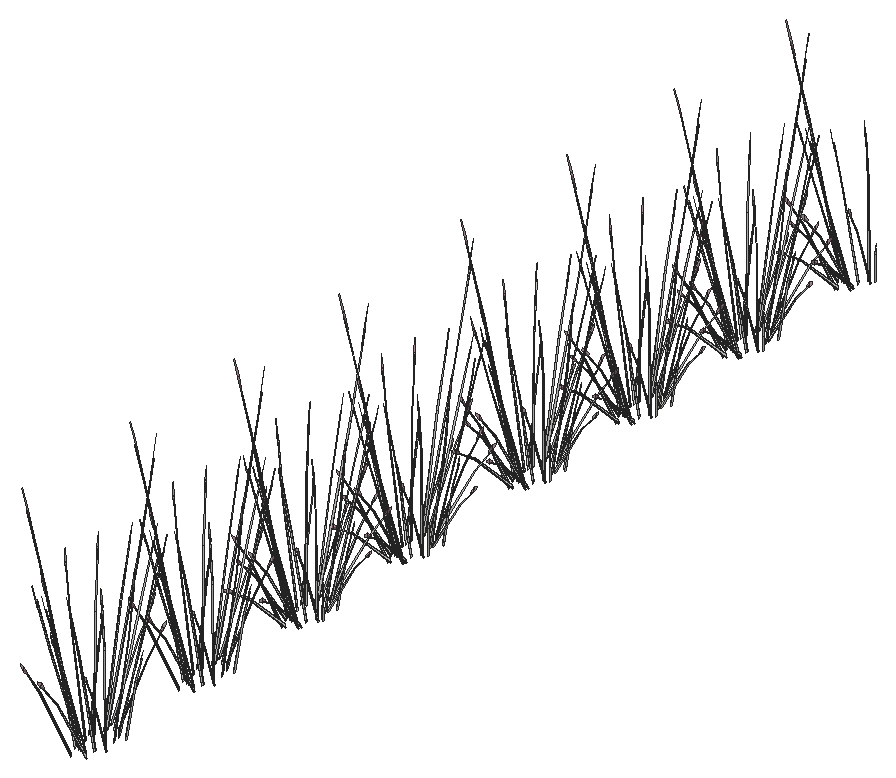
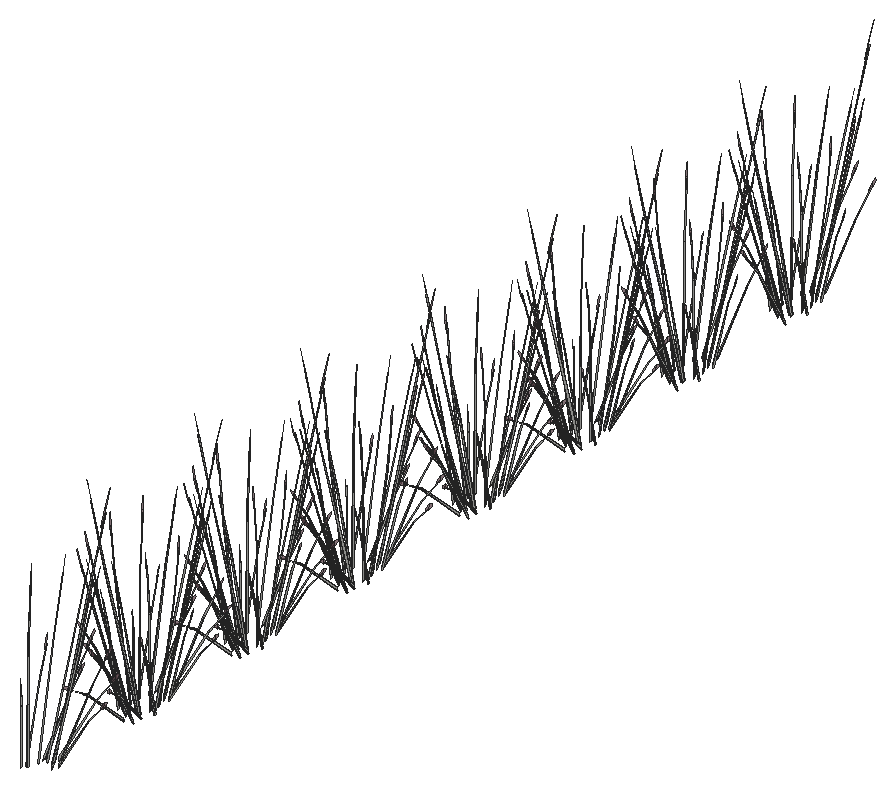
# SketchUp Ruby script. Lengths in inches.
U = 1.inch
M = Sketchup.active_model
def pt(a) = Geom::Point3d.new(a.map { |v| v * U })
def face(e, loops, mat)
  f = e.add_face(loops[0].map { |a| pt(a) })
  loops[1..].each { |l| e.add_face(l.map { |a| pt(a) }).erase! }
  f.material = f.back_material = mat if mat
  f
end
# faces: each face lists its corners as indices into pts; further lists are holes
def faces(e, pts, list, mat = nil) = list.each { |f| face(e, (f[0].is_a?(Array) ? f : [f]).map { |l| l.map { |i| pts[i] } }, mat) }
# xy, xz, yz: faces in a plane at the given z, y or x. An outline is a flat list of corners, or four numbers for a rectangle; further outlines are holes
def ring(l) = l.size == 4 ? [[l[0], l[1]], [l[2], l[1]], [l[2], l[3]], [l[0], l[3]]] : l.each_slice(2).to_a
def flat(e, list, mat, &to3) = list.each { |f| face(e, (f[0].is_a?(Array) ? f : [f]).map { |l| ring(l).map { |u, v| to3.(u, v) } }, mat) }
def xy(e, z, list, mat = nil) = flat(e, list, mat) { |x, y| [x, y, z] }
def xz(e, y, list, mat = nil) = flat(e, list, mat) { |x, z| [x, y, z] }
def yz(e, x, list, mat = nil) = flat(e, list, mat) { |y, z| [x, y, z] }
def lines(e, pts, list) = list.each { |a, b| e.add_line(pt(pts[a]), pt(pts[b])) }
# prism: a flat outline (further loops are holes) pulled along v
def prism(e, loops, v, mat = nil)
  f = face(e, loops, mat); d = Geom::Vector3d.new(v.map { |x| x * U })
  f.pushpull(f.normal.samedirection?(d) ? d.length : -d.length)
end
def box(e, o, s, mat = nil) = prism(e, [[o, [o[0] + s[0], o[1], o[2]], [o[0] + s[0], o[1] + s[1], o[2]], [o[0], o[1] + s[1], o[2]]]], [0, 0, s[2]], mat)
def at(x, y, z, deg = 0) = Geom::Transformation.translation(pt([x, y, z])) * Geom::Transformation.rotation(ORIGIN, Z_AXIS, deg.degrees)
def axes(o, x, y, z) = Geom::Transformation.new([*x, 0, *y, 0, *z, 0, *pt(o).to_a, 1])
def part(name) = M.definitions.add(name)
# library, detail: a bought-in or finely detailed component or shape, given as its bounding box
def library(name, o, s) = part(name).tap { |d| box(d.entities, o, s) }
def detail(e, o, s) = box(e.add_group.entities, o, s)
def put(e, d, t, mat = nil) = e.add_instance(d, t).tap { |i| i.material = mat if mat }
def group(e, t, mat = nil) = e.add_group.tap { |g| g.transformation = t; g.material = mat if mat }.entities
root = M.entities
M.materials.add("LightPink_Translucent").color = [144, 107, 117]
M.materials["LightPink_Translucent"].alpha = 0.75
c1 = part("blade")
p = [[2.15,0.21,22],[0,0.17,0],[0.09,0.45,0],[2.18,0.31,22],[2.29,0.31,22],[0.38,0.45,0],
  [2.48,0.24,33],[2.49,0.24,33],[2.48,0.22,33]]
faces(c1.entities,p,[[0,1,2,3],[4,5,2,3],[6,3,4,7],[8,0,3,6]])
c2 = part("seeds")
p = [[0.3,-0.1,1.38],[-0.01,-0.03,1.59],[-0.01,-0.03,0.03],[0.14,-0.07,-0.07],[0.29,-0.03,3],[0.15,0.01,3.11]]
faces(c2.entities,p,[[0,1,2,3],[1,0,4,5]],"LightPink_Translucent")
c3 = part("blade with seeds")
put(c3.entities,c1,at(0,0,0))
put(c3.entities,c2,axes([2.4,0.25,30.99],[1.5799,-0.05474,1.17369],[-0.12525,1.92788,0.29478],[-0.07173,-0.02425,1.56792]))
put(root,c3,axes([252.66,9.92,2.61],[-0.02599,0.0467,1.28742],[-0.25468,-0.15757,-0.12165],[-0.00922,-0.20381,0.22783]))
put(root,c3,axes([251.28,9.02,2.61],[-0.00478,0.07329,1.28742],[-0.23551,0.26599,-0.12165],[-0.0693,-0.13596,0.22783]))
put(root,c3,axes([251.9375,10.4,2.625],[0.1886,-0.20781,0.04667],[0.09231,0.37894,0.3674],[-0.01821,-0.16704,0.56022]))
put(root,c3,axes([251.29,10.46,2.625],[0.11633,-0.38842,0.04667],[0.16566,0.22614,0.3674],[-0.05356,-0.12453,0.56022]))
put(root,c3,axes([251.34,10.41,3.13],[-0.17082,0.58618,-0.09885],[-0.24738,-0.33771,-0.54865],[-0.08599,-0.16561,0.83366]))
put(root,c3,axes([252.51,11.0625,2.625],[0.21034,0.02849,0.04667],[-0.00577,0.43021,0.3674],[0.02201,-0.1648,0.56022]))
put(root,c3,axes([253.35,12.25,2.61],[-0.03343,-0.00464,1.28742],[-0.13883,-0.49759,-0.12165],[0.05575,-0.16361,0.22783]))
put(root,c3,axes([250.75,11.22,2.625],[0.01289,-0.46496,0.04667],[0.19462,0.01275,0.3674],[-0.07455,-0.04865,0.56022]))
put(root,c3,axes([252.86,12.27,2.625],[0.17571,0.25715,0.04667],[-0.1023,0.3662,0.3674],[0.05634,-0.11839,0.56022]))
put(root,c3,axes([250.48,10.61,2.61],[0.01898,0.06102,1.28742],[-0.09148,0.54852,-0.12165],[-0.09264,0.00397,0.22783]))
put(root,c3,axes([250.44,12.49,2.625],[-0.09401,-0.41691,0.04667],[0.17143,-0.20406,0.3674],[-0.07557,0.04026,0.56022]))
put(root,c3,axes([252.88,13.7,2.625],[0.09401,0.41691,0.04667],[-0.17143,0.20406,0.3674],[0.07557,-0.04026,0.56022]))
put(root,c3,axes([253.29,15.35,2.61],[-0.02314,-0.05353,1.28742],[0.05063,-0.5738,-0.12165],[0.09117,-0.03666,0.22783]))
put(root,c3,axes([250.47,13.91,2.625],[-0.17571,-0.25715,0.04667],[0.1023,-0.3662,0.3674],[-0.05634,0.11839,0.56022]))
put(root,c3,axes([249.81,13.61,2.61],[0.03267,0.0164,1.28742],[0.10105,0.54025,-0.12165],[-0.06687,0.1418,0.22783]))
put(root,c3,axes([252.58,14.96,2.625],[-0.01289,0.46496,0.04667],[-0.19462,-0.01275,0.3674],[0.07455,0.04865,0.56022]))
put(root,c3,axes([251.78,15.97,2.61],[0.00076,-0.07403,1.28742],[0.21935,-0.3266,-0.12165],[0.07619,0.11658,0.22783]))
put(root,c3,axes([250.82,15.12,2.625],[-0.21034,-0.02849,0.04667],[0.00577,-0.43021,0.3674],[-0.02201,0.1648,0.56022]))
put(root,c3,axes([252.04,15.73,2.625],[-0.11633,0.38842,0.04667],[-0.16566,-0.22614,0.3674],[0.05356,0.12453,0.56022]))
put(root,c3,axes([251.39,15.79,2.625],[-0.1886,0.20781,0.04667],[-0.09231,-0.37894,0.3674],[0.01821,0.16704,0.56022]))
put(root,c3,axes([250.86,14.92,3.11],[0.2813,0.0303,-0.09797],[-0.00769,0.57361,-0.54375],[-0.01954,0.22092,0.82622]))
put(root,c3,axes([250.27,16.43,2.61],[0.02904,-0.03692,1.28742],[0.24001,0.24555,-0.12165],[-0.00564,0.20445,0.22783]))
put(root,c3,axes([252.66,26.78,2.61],[-0.02599,0.0467,1.28742],[-0.25468,-0.15757,-0.12165],[-0.00922,-0.20381,0.22783]))
put(root,c3,axes([251.28,25.89,2.61],[-0.00478,0.07329,1.28742],[-0.23551,0.26599,-0.12165],[-0.0693,-0.13596,0.22783]))
put(root,c3,axes([251.9375,27.27,2.625],[0.1886,-0.20781,0.04667],[0.09231,0.37894,0.3674],[-0.01821,-0.16704,0.56022]))
put(root,c3,axes([251.29,27.32,2.625],[0.11633,-0.38842,0.04667],[0.16566,0.22614,0.3674],[-0.05356,-0.12453,0.56022]))
put(root,c3,axes([251.34,27.28,3.13],[-0.17082,0.58618,-0.09885],[-0.24738,-0.33771,-0.54865],[-0.08599,-0.16561,0.83366]))
put(root,c3,axes([252.51,27.93,2.625],[0.21034,0.02849,0.04667],[-0.00577,0.43021,0.3674],[0.02201,-0.1648,0.56022]))
put(root,c3,axes([253.35,29.12,2.61],[-0.03343,-0.00464,1.28742],[-0.13883,-0.49759,-0.12165],[0.05575,-0.16361,0.22783]))
put(root,c3,axes([250.75,28.09,2.625],[0.01289,-0.46496,0.04667],[0.19462,0.01275,0.3674],[-0.07455,-0.04865,0.56022]))
put(root,c3,axes([252.86,29.14,2.625],[0.17571,0.25715,0.04667],[-0.1023,0.3662,0.3674],[0.05634,-0.11839,0.56022]))
put(root,c3,axes([250.48,27.48,2.61],[0.01898,0.06102,1.28742],[-0.09148,0.54852,-0.12165],[-0.09264,0.00397,0.22783]))
put(root,c3,axes([250.44,29.35,2.625],[-0.09401,-0.41691,0.04667],[0.17143,-0.20406,0.3674],[-0.07557,0.04026,0.56022]))
put(root,c3,axes([252.88,30.57,2.625],[0.09401,0.41691,0.04667],[-0.17143,0.20406,0.3674],[0.07557,-0.04026,0.56022]))
put(root,c3,axes([253.29,32.22,2.61],[-0.02314,-0.05353,1.28742],[0.05063,-0.5738,-0.12165],[0.09117,-0.03666,0.22783]))
put(root,c3,axes([250.47,30.78,2.625],[-0.17571,-0.25715,0.04667],[0.1023,-0.3662,0.3674],[-0.05634,0.11839,0.56022]))
put(root,c3,axes([249.81,30.48,2.61],[0.03267,0.0164,1.28742],[0.10105,0.54025,-0.12165],[-0.06687,0.1418,0.22783]))
put(root,c3,axes([252.58,31.83,2.625],[-0.01289,0.46496,0.04667],[-0.19462,-0.01275,0.3674],[0.07455,0.04865,0.56022]))
put(root,c3,axes([251.78,32.84,2.61],[0.00076,-0.07403,1.28742],[0.21935,-0.3266,-0.12165],[0.07619,0.11658,0.22783]))
put(root,c3,axes([250.82,31.99,2.625],[-0.21034,-0.02849,0.04667],[0.00577,-0.43021,0.3674],[-0.02201,0.1648,0.56022]))
put(root,c3,axes([252.04,32.6,2.625],[-0.11633,0.38842,0.04667],[-0.16566,-0.22614,0.3674],[0.05356,0.12453,0.56022]))
put(root,c3,axes([251.39,32.65,2.625],[-0.1886,0.20781,0.04667],[-0.09231,-0.37894,0.3674],[0.01821,0.16704,0.56022]))
put(root,c3,axes([250.86,31.79,3.11],[0.2813,0.0303,-0.09797],[-0.00769,0.57361,-0.54375],[-0.01954,0.22092,0.82622]))
put(root,c3,axes([250.27,33.3,2.61],[0.02904,-0.03692,1.28742],[0.24001,0.24555,-0.12165],[-0.00564,0.20445,0.22783]))
put(root,c3,axes([251.55,42.32,2.61],[-0.03915,-0.08573,1.26972],[-0.26126,0.05435,-0.2008],[-0.0417,-0.20505,0.10183]))
put(root,c3,axes([252.72,43.375,2.61],[-0.00247,-0.12169,1.26972],[-0.20868,-0.35171,-0.2008],[0.03226,-0.2132,0.10183]))
put(root,c3,axes([252.66,42.9375,2.61],[-0.02599,0.0467,1.28742],[-0.25468,-0.15757,-0.12165],[-0.00922,-0.20381,0.22783]))
put(root,c3,axes([251.28,42.04,2.61],[-0.00478,0.07329,1.28742],[-0.23551,0.26599,-0.12165],[-0.0693,-0.13596,0.22783]))
put(root,c3,axes([251.9375,43.42,2.625],[0.1886,-0.20781,0.04667],[0.09231,0.37894,0.3674],[-0.01821,-0.16704,0.56022]))
put(root,c3,axes([251.29,43.48,2.625],[0.11633,-0.38842,0.04667],[0.16566,0.22614,0.3674],[-0.05356,-0.12453,0.56022]))
put(root,c3,axes([251.34,43.44,3.13],[-0.17082,0.58618,-0.09885],[-0.24738,-0.33771,-0.54865],[-0.08599,-0.16561,0.83366]))
put(root,c3,axes([252.51,44.08,2.625],[0.21034,0.02849,0.04667],[-0.00577,0.43021,0.3674],[0.02201,-0.1648,0.56022]))
put(root,c3,axes([250.6875,43.27,2.61],[-0.05507,-0.00432,1.26972],[-0.17533,0.4316,-0.2008],[-0.09355,-0.08819,0.10183]))
put(root,c3,axes([253.35,45.27,2.61],[-0.03343,-0.00464,1.28742],[-0.13883,-0.49759,-0.12165],[0.05575,-0.16361,0.22783]))
put(root,c3,axes([250.75,44.24,2.625],[0.01289,-0.46496,0.04667],[0.19462,0.01275,0.3674],[-0.07455,-0.04865,0.56022]))
put(root,c3,axes([252.86,45.29,2.625],[0.17571,0.25715,0.04667],[-0.1023,0.3662,0.3674],[0.05634,-0.11839,0.56022]))
put(root,c3,axes([253.48,45.86,2.61],[0.03552,-0.09314,1.26972],[-0.04546,-0.57131,-0.2008],[0.08912,-0.10832,0.10183]))
put(root,c3,axes([250.48,43.63,2.61],[0.01898,0.06102,1.28742],[-0.09148,0.54852,-0.12165],[-0.09264,0.00397,0.22783]))
put(root,c3,axes([250.44,45.51,2.625],[-0.09401,-0.41691,0.04667],[0.17143,-0.20406,0.3674],[-0.07557,0.04026,0.56022]))
put(root,c3,axes([252.88,46.72,2.625],[0.09401,0.41691,0.04667],[-0.17143,0.20406,0.3674],[0.07557,-0.04026,0.56022]))
put(root,c3,axes([253.29,48.375,2.61],[-0.02314,-0.05353,1.28742],[0.05063,-0.5738,-0.12165],[0.09117,-0.03666,0.22783]))
put(root,c3,axes([252.72,47.51,2.61],[0.05491,-0.01034,1.26972],[0.1506,-0.47504,-0.2008],[0.09767,0.06271,0.10183]))
put(root,c3,axes([250.47,46.93,2.625],[-0.17571,-0.25715,0.04667],[0.1023,-0.3662,0.3674],[-0.05634,0.11839,0.56022]))
put(root,c3,axes([249.81,46.63,2.61],[0.03267,0.0164,1.28742],[0.10105,0.54025,-0.12165],[-0.06687,0.1418,0.22783]))
put(root,c3,axes([252.58,47.98,2.625],[-0.01289,0.46496,0.04667],[-0.19462,-0.01275,0.3674],[0.07455,0.04865,0.56022]))
put(root,c3,axes([251.78,48.99,2.61],[0.00076,-0.07403,1.28742],[0.21935,-0.3266,-0.12165],[0.07619,0.11658,0.22783]))
put(root,c3,axes([250.82,48.14,2.625],[-0.21034,-0.02849,0.04667],[0.00577,-0.43021,0.3674],[-0.02201,0.1648,0.56022]))
put(root,c3,axes([252.04,48.75,2.625],[-0.11633,0.38842,0.04667],[-0.16566,-0.22614,0.3674],[0.05356,0.12453,0.56022]))
put(root,c3,axes([251.39,48.81,2.625],[-0.1886,0.20781,0.04667],[-0.09231,-0.37894,0.3674],[0.01821,0.16704,0.56022]))
put(root,c3,axes([250.29,48.21,2.61],[-0.00636,0.121,1.26972],[0.18056,0.42094,-0.2008],[-0.04727,0.19906,0.10183]))
put(root,c3,axes([250.86,47.9375,3.11],[0.2813,0.0303,-0.09797],[-0.00769,0.57361,-0.54375],[-0.01954,0.22092,0.82622]))
put(root,c3,axes([250.27,49.45,2.61],[0.02904,-0.03692,1.28742],[0.24001,0.24555,-0.12165],[-0.00564,0.20445,0.22783]))
put(root,c3,axes([251.32,49.71,2.61],[0.03244,0.09846,1.26972],[0.26183,0.03868,-0.2008],[0.02633,0.21715,0.10183]))
put(root,c3,axes([251.55,58.77,2.61],[-0.03915,-0.08573,1.26972],[-0.26126,0.05435,-0.2008],[-0.0417,-0.20505,0.10183]))
put(root,c3,axes([252.72,59.82,2.61],[-0.00247,-0.12169,1.26972],[-0.20868,-0.35171,-0.2008],[0.03226,-0.2132,0.10183]))
put(root,c3,axes([252.66,59.39,2.61],[-0.02599,0.0467,1.28742],[-0.25468,-0.15757,-0.12165],[-0.00922,-0.20381,0.22783]))
put(root,c3,axes([251.28,58.49,2.61],[-0.00478,0.07329,1.28742],[-0.23551,0.26599,-0.12165],[-0.0693,-0.13596,0.22783]))
put(root,c3,axes([251.9375,59.87,2.625],[0.1886,-0.20781,0.04667],[0.09231,0.37894,0.3674],[-0.01821,-0.16704,0.56022]))
put(root,c3,axes([251.29,59.93,2.625],[0.11633,-0.38842,0.04667],[0.16566,0.22614,0.3674],[-0.05356,-0.12453,0.56022]))
put(root,c3,axes([251.34,59.89,3.13],[-0.17082,0.58618,-0.09885],[-0.24738,-0.33771,-0.54865],[-0.08599,-0.16561,0.83366]))
put(root,c3,axes([252.51,60.53,2.625],[0.21034,0.02849,0.04667],[-0.00577,0.43021,0.3674],[0.02201,-0.1648,0.56022]))
put(root,c3,axes([250.6875,59.72,2.61],[-0.05507,-0.00432,1.26972],[-0.17533,0.4316,-0.2008],[-0.09355,-0.08819,0.10183]))
put(root,c3,axes([253.35,61.72,2.61],[-0.03343,-0.00464,1.28742],[-0.13883,-0.49759,-0.12165],[0.05575,-0.16361,0.22783]))
put(root,c3,axes([250.75,60.69,2.625],[0.01289,-0.46496,0.04667],[0.19462,0.01275,0.3674],[-0.07455,-0.04865,0.56022]))
put(root,c3,axes([252.86,61.74,2.625],[0.17571,0.25715,0.04667],[-0.1023,0.3662,0.3674],[0.05634,-0.11839,0.56022]))
put(root,c3,axes([253.48,62.3125,2.61],[0.03552,-0.09314,1.26972],[-0.04546,-0.57131,-0.2008],[0.08912,-0.10832,0.10183]))
put(root,c3,axes([250.48,60.08,2.61],[0.01898,0.06102,1.28742],[-0.09148,0.54852,-0.12165],[-0.09264,0.00397,0.22783]))
put(root,c3,axes([250.44,61.96,2.625],[-0.09401,-0.41691,0.04667],[0.17143,-0.20406,0.3674],[-0.07557,0.04026,0.56022]))
put(root,c3,axes([252.88,63.17,2.625],[0.09401,0.41691,0.04667],[-0.17143,0.20406,0.3674],[0.07557,-0.04026,0.56022]))
put(root,c3,axes([253.29,64.83,2.61],[-0.02314,-0.05353,1.28742],[0.05063,-0.5738,-0.12165],[0.09117,-0.03666,0.22783]))
put(root,c3,axes([250.28,62.5,2.61],[-0.0418,0.07939,1.26972],[0.00356,0.58003,-0.2008],[-0.09581,0.07543,0.10183]))
put(root,c3,axes([252.72,63.96,2.61],[0.05491,-0.01034,1.26972],[0.1506,-0.47504,-0.2008],[0.09767,0.06271,0.10183]))
put(root,c3,axes([250.47,63.39,2.625],[-0.17571,-0.25715,0.04667],[0.1023,-0.3662,0.3674],[-0.05634,0.11839,0.56022]))
put(root,c3,axes([249.81,63.08,2.61],[0.03267,0.0164,1.28742],[0.10105,0.54025,-0.12165],[-0.06687,0.1418,0.22783]))
put(root,c3,axes([252.58,64.43,2.625],[-0.01289,0.46496,0.04667],[-0.19462,-0.01275,0.3674],[0.07455,0.04865,0.56022]))
put(root,c3,axes([251.78,65.44,2.61],[0.00076,-0.07403,1.28742],[0.21935,-0.3266,-0.12165],[0.07619,0.11658,0.22783]))
put(root,c3,axes([250.82,64.59,2.625],[-0.21034,-0.02849,0.04667],[0.00577,-0.43021,0.3674],[-0.02201,0.1648,0.56022]))
put(root,c3,axes([252.04,65.2,2.625],[-0.11633,0.38842,0.04667],[-0.16566,-0.22614,0.3674],[0.05356,0.12453,0.56022]))
put(root,c3,axes([251.39,65.26,2.625],[-0.1886,0.20781,0.04667],[-0.09231,-0.37894,0.3674],[0.01821,0.16704,0.56022]))
put(root,c3,axes([250.29,64.66,2.61],[-0.00636,0.121,1.26972],[0.18056,0.42094,-0.2008],[-0.04727,0.19906,0.10183]))
put(root,c3,axes([250.86,64.39,3.11],[0.2813,0.0303,-0.09797],[-0.00769,0.57361,-0.54375],[-0.01954,0.22092,0.82622]))
put(root,c3,axes([250.27,65.9,2.61],[0.02904,-0.03692,1.28742],[0.24001,0.24555,-0.12165],[-0.00564,0.20445,0.22783]))
put(root,c3,axes([251.32,66.16,2.61],[0.03244,0.09846,1.26972],[0.26183,0.03868,-0.2008],[0.02633,0.21715,0.10183]))
put(root,c3,axes([251.55,77.8,2.61],[-0.03915,-0.08573,1.26972],[-0.26126,0.05435,-0.2008],[-0.0417,-0.20505,0.10183]))
put(root,c3,axes([252.72,78.85,2.61],[-0.00247,-0.12169,1.26972],[-0.20868,-0.35171,-0.2008],[0.03226,-0.2132,0.10183]))
put(root,c3,axes([252.66,78.41,2.61],[-0.02599,0.0467,1.28742],[-0.25468,-0.15757,-0.12165],[-0.00922,-0.20381,0.22783]))
put(root,c3,axes([251.28,77.52,2.61],[-0.00478,0.07329,1.28742],[-0.23551,0.26599,-0.12165],[-0.0693,-0.13596,0.22783]))
put(root,c3,axes([251.9375,78.89,2.625],[0.1886,-0.20781,0.04667],[0.09231,0.37894,0.3674],[-0.01821,-0.16704,0.56022]))
put(root,c3,axes([251.29,78.95,2.625],[0.11633,-0.38842,0.04667],[0.16566,0.22614,0.3674],[-0.05356,-0.12453,0.56022]))
put(root,c3,axes([251.34,78.91,3.13],[-0.17082,0.58618,-0.09885],[-0.24738,-0.33771,-0.54865],[-0.08599,-0.16561,0.83366]))
put(root,c3,axes([252.51,79.56,2.625],[0.21034,0.02849,0.04667],[-0.00577,0.43021,0.3674],[0.02201,-0.1648,0.56022]))
put(root,c3,axes([250.6875,78.74,2.61],[-0.05507,-0.00432,1.26972],[-0.17533,0.4316,-0.2008],[-0.09355,-0.08819,0.10183]))
put(root,c3,axes([253.35,80.74,2.61],[-0.03343,-0.00464,1.28742],[-0.13883,-0.49759,-0.12165],[0.05575,-0.16361,0.22783]))
put(root,c3,axes([250.75,79.72,2.625],[0.01289,-0.46496,0.04667],[0.19462,0.01275,0.3674],[-0.07455,-0.04865,0.56022]))
put(root,c3,axes([252.86,80.76,2.625],[0.17571,0.25715,0.04667],[-0.1023,0.3662,0.3674],[0.05634,-0.11839,0.56022]))
put(root,c3,axes([253.48,81.34,2.61],[0.03552,-0.09314,1.26972],[-0.04546,-0.57131,-0.2008],[0.08912,-0.10832,0.10183]))
put(root,c3,axes([250.48,79.11,2.61],[0.01898,0.06102,1.28742],[-0.09148,0.54852,-0.12165],[-0.09264,0.00397,0.22783]))
put(root,c3,axes([250.44,80.98,2.625],[-0.09401,-0.41691,0.04667],[0.17143,-0.20406,0.3674],[-0.07557,0.04026,0.56022]))
put(root,c3,axes([252.88,82.19,2.625],[0.09401,0.41691,0.04667],[-0.17143,0.20406,0.3674],[0.07557,-0.04026,0.56022]))
put(root,c3,axes([253.29,83.85,2.61],[-0.02314,-0.05353,1.28742],[0.05063,-0.5738,-0.12165],[0.09117,-0.03666,0.22783]))
put(root,c3,axes([250.28,81.52,2.61],[-0.0418,0.07939,1.26972],[0.00356,0.58003,-0.2008],[-0.09581,0.07543,0.10183]))
put(root,c3,axes([252.72,82.98,2.61],[0.05491,-0.01034,1.26972],[0.1506,-0.47504,-0.2008],[0.09767,0.06271,0.10183]))
put(root,c3,axes([250.47,82.41,2.625],[-0.17571,-0.25715,0.04667],[0.1023,-0.3662,0.3674],[-0.05634,0.11839,0.56022]))
put(root,c3,axes([249.81,82.11,2.61],[0.03267,0.0164,1.28742],[0.10105,0.54025,-0.12165],[-0.06687,0.1418,0.22783]))
put(root,c3,axes([252.58,83.46,2.625],[-0.01289,0.46496,0.04667],[-0.19462,-0.01275,0.3674],[0.07455,0.04865,0.56022]))
put(root,c3,axes([251.78,84.47,2.61],[0.00076,-0.07403,1.28742],[0.21935,-0.3266,-0.12165],[0.07619,0.11658,0.22783]))
put(root,c3,axes([250.82,83.62,2.625],[-0.21034,-0.02849,0.04667],[0.00577,-0.43021,0.3674],[-0.02201,0.1648,0.56022]))
put(root,c3,axes([252.04,84.22,2.625],[-0.11633,0.38842,0.04667],[-0.16566,-0.22614,0.3674],[0.05356,0.12453,0.56022]))
put(root,c3,axes([251.39,84.28,2.625],[-0.1886,0.20781,0.04667],[-0.09231,-0.37894,0.3674],[0.01821,0.16704,0.56022]))
put(root,c3,axes([250.29,83.6875,2.61],[-0.00636,0.121,1.26972],[0.18056,0.42094,-0.2008],[-0.04727,0.19906,0.10183]))
put(root,c3,axes([250.86,83.41,3.11],[0.2813,0.0303,-0.09797],[-0.00769,0.57361,-0.54375],[-0.01954,0.22092,0.82622]))
put(root,c3,axes([250.27,84.93,2.61],[0.02904,-0.03692,1.28742],[0.24001,0.24555,-0.12165],[-0.00564,0.20445,0.22783]))
put(root,c3,axes([251.32,85.18,2.61],[0.03244,0.09846,1.26972],[0.26183,0.03868,-0.2008],[0.02633,0.21715,0.10183]))
put(root,c3,axes([251.55,94.375,2.61],[-0.03915,-0.08573,1.26972],[-0.26126,0.05435,-0.2008],[-0.0417,-0.20505,0.10183]))
put(root,c3,axes([252.72,95.43,2.61],[-0.00247,-0.12169,1.26972],[-0.20868,-0.35171,-0.2008],[0.03226,-0.2132,0.10183]))
put(root,c3,axes([252.66,94.99,2.61],[-0.02599,0.0467,1.28742],[-0.25468,-0.15757,-0.12165],[-0.00922,-0.20381,0.22783]))
put(root,c3,axes([251.28,94.09,2.61],[-0.00478,0.07329,1.28742],[-0.23551,0.26599,-0.12165],[-0.0693,-0.13596,0.22783]))
put(root,c3,axes([251.9375,95.47,2.625],[0.1886,-0.20781,0.04667],[0.09231,0.37894,0.3674],[-0.01821,-0.16704,0.56022]))
put(root,c3,axes([251.29,95.53,2.625],[0.11633,-0.38842,0.04667],[0.16566,0.22614,0.3674],[-0.05356,-0.12453,0.56022]))
put(root,c3,axes([251.34,95.49,3.13],[-0.17082,0.58618,-0.09885],[-0.24738,-0.33771,-0.54865],[-0.08599,-0.16561,0.83366]))
put(root,c3,axes([252.51,96.13,2.625],[0.21034,0.02849,0.04667],[-0.00577,0.43021,0.3674],[0.02201,-0.1648,0.56022]))
put(root,c3,axes([250.6875,95.32,2.61],[-0.05507,-0.00432,1.26972],[-0.17533,0.4316,-0.2008],[-0.09355,-0.08819,0.10183]))
put(root,c3,axes([253.35,97.32,2.61],[-0.03343,-0.00464,1.28742],[-0.13883,-0.49759,-0.12165],[0.05575,-0.16361,0.22783]))
put(root,c3,axes([250.75,96.29,2.625],[0.01289,-0.46496,0.04667],[0.19462,0.01275,0.3674],[-0.07455,-0.04865,0.56022]))
put(root,c3,axes([252.86,97.34,2.625],[0.17571,0.25715,0.04667],[-0.1023,0.3662,0.3674],[0.05634,-0.11839,0.56022]))
put(root,c3,axes([253.48,97.91,2.61],[0.03552,-0.09314,1.26972],[-0.04546,-0.57131,-0.2008],[0.08912,-0.10832,0.10183]))
put(root,c3,axes([250.48,95.69,2.61],[0.01898,0.06102,1.28742],[-0.09148,0.54852,-0.12165],[-0.09264,0.00397,0.22783]))
put(root,c3,axes([250.44,97.56,2.625],[-0.09401,-0.41691,0.04667],[0.17143,-0.20406,0.3674],[-0.07557,0.04026,0.56022]))
put(root,c3,axes([252.88,98.77,2.625],[0.09401,0.41691,0.04667],[-0.17143,0.20406,0.3674],[0.07557,-0.04026,0.56022]))
put(root,c3,axes([253.29,100.43,2.61],[-0.02314,-0.05353,1.28742],[0.05063,-0.5738,-0.12165],[0.09117,-0.03666,0.22783]))
put(root,c3,axes([250.28,98.1,2.61],[-0.0418,0.07939,1.26972],[0.00356,0.58003,-0.2008],[-0.09581,0.07543,0.10183]))
put(root,c3,axes([252.72,99.56,2.61],[0.05491,-0.01034,1.26972],[0.1506,-0.47504,-0.2008],[0.09767,0.06271,0.10183]))
put(root,c3,axes([250.47,98.99,2.625],[-0.17571,-0.25715,0.04667],[0.1023,-0.3662,0.3674],[-0.05634,0.11839,0.56022]))
put(root,c3,axes([249.81,98.6875,2.61],[0.03267,0.0164,1.28742],[0.10105,0.54025,-0.12165],[-0.06687,0.1418,0.22783]))
put(root,c3,axes([252.58,100.04,2.625],[-0.01289,0.46496,0.04667],[-0.19462,-0.01275,0.3674],[0.07455,0.04865,0.56022]))
put(root,c3,axes([251.78,101.04,2.61],[0.00076,-0.07403,1.28742],[0.21935,-0.3266,-0.12165],[0.07619,0.11658,0.22783]))
put(root,c3,axes([250.82,100.19,2.625],[-0.21034,-0.02849,0.04667],[0.00577,-0.43021,0.3674],[-0.02201,0.1648,0.56022]))
put(root,c3,axes([252.04,100.8,2.625],[-0.11633,0.38842,0.04667],[-0.16566,-0.22614,0.3674],[0.05356,0.12453,0.56022]))
put(root,c3,axes([251.39,100.86,2.625],[-0.1886,0.20781,0.04667],[-0.09231,-0.37894,0.3674],[0.01821,0.16704,0.56022]))
put(root,c3,axes([250.29,100.26,2.61],[-0.00636,0.121,1.26972],[0.18056,0.42094,-0.2008],[-0.04727,0.19906,0.10183]))
put(root,c3,axes([250.86,99.99,3.11],[0.2813,0.0303,-0.09797],[-0.00769,0.57361,-0.54375],[-0.01954,0.22092,0.82622]))
put(root,c3,axes([250.27,101.5,2.61],[0.02904,-0.03692,1.28742],[0.24001,0.24555,-0.12165],[-0.00564,0.20445,0.22783]))
put(root,c3,axes([251.32,101.76,2.61],[0.03244,0.09846,1.26972],[0.26183,0.03868,-0.2008],[0.02633,0.21715,0.10183]))
put(root,c3,axes([251.55,111.13,2.61],[-0.03915,-0.08573,1.26972],[-0.26126,0.05435,-0.2008],[-0.0417,-0.20505,0.10183]))
put(root,c3,axes([252.72,112.18,2.61],[-0.00247,-0.12169,1.26972],[-0.20868,-0.35171,-0.2008],[0.03226,-0.2132,0.10183]))
put(root,c3,axes([252.66,111.74,2.61],[-0.02599,0.0467,1.28742],[-0.25468,-0.15757,-0.12165],[-0.00922,-0.20381,0.22783]))
put(root,c3,axes([251.28,110.85,2.61],[-0.00478,0.07329,1.28742],[-0.23551,0.26599,-0.12165],[-0.0693,-0.13596,0.22783]))
put(root,c3,axes([251.9375,112.23,2.625],[0.1886,-0.20781,0.04667],[0.09231,0.37894,0.3674],[-0.01821,-0.16704,0.56022]))
put(root,c3,axes([251.29,112.28,2.625],[0.11633,-0.38842,0.04667],[0.16566,0.22614,0.3674],[-0.05356,-0.12453,0.56022]))
put(root,c3,axes([251.34,112.24,3.13],[-0.17082,0.58618,-0.09885],[-0.24738,-0.33771,-0.54865],[-0.08599,-0.16561,0.83366]))
put(root,c3,axes([252.51,112.89,2.625],[0.21034,0.02849,0.04667],[-0.00577,0.43021,0.3674],[0.02201,-0.1648,0.56022]))
put(root,c3,axes([250.6875,112.07,2.61],[-0.05507,-0.00432,1.26972],[-0.17533,0.4316,-0.2008],[-0.09355,-0.08819,0.10183]))
put(root,c3,axes([253.35,114.08,2.61],[-0.03343,-0.00464,1.28742],[-0.13883,-0.49759,-0.12165],[0.05575,-0.16361,0.22783]))
put(root,c3,axes([250.75,113.05,2.625],[0.01289,-0.46496,0.04667],[0.19462,0.01275,0.3674],[-0.07455,-0.04865,0.56022]))
put(root,c3,axes([252.86,114.1,2.625],[0.17571,0.25715,0.04667],[-0.1023,0.3662,0.3674],[0.05634,-0.11839,0.56022]))
put(root,c3,axes([253.48,114.67,2.61],[0.03552,-0.09314,1.26972],[-0.04546,-0.57131,-0.2008],[0.08912,-0.10832,0.10183]))
put(root,c3,axes([250.48,112.44,2.61],[0.01898,0.06102,1.28742],[-0.09148,0.54852,-0.12165],[-0.09264,0.00397,0.22783]))
put(root,c3,axes([250.44,114.3125,2.625],[-0.09401,-0.41691,0.04667],[0.17143,-0.20406,0.3674],[-0.07557,0.04026,0.56022]))
put(root,c3,axes([252.88,115.53,2.625],[0.09401,0.41691,0.04667],[-0.17143,0.20406,0.3674],[0.07557,-0.04026,0.56022]))
put(root,c3,axes([253.29,117.18,2.61],[-0.02314,-0.05353,1.28742],[0.05063,-0.5738,-0.12165],[0.09117,-0.03666,0.22783]))
put(root,c3,axes([250.28,114.85,2.61],[-0.0418,0.07939,1.26972],[0.00356,0.58003,-0.2008],[-0.09581,0.07543,0.10183]))
put(root,c3,axes([252.72,116.31,2.61],[0.05491,-0.01034,1.26972],[0.1506,-0.47504,-0.2008],[0.09767,0.06271,0.10183]))
put(root,c3,axes([250.47,115.74,2.625],[-0.17571,-0.25715,0.04667],[0.1023,-0.3662,0.3674],[-0.05634,0.11839,0.56022]))
put(root,c3,axes([249.81,115.44,2.61],[0.03267,0.0164,1.28742],[0.10105,0.54025,-0.12165],[-0.06687,0.1418,0.22783]))
put(root,c3,axes([252.58,116.79,2.625],[-0.01289,0.46496,0.04667],[-0.19462,-0.01275,0.3674],[0.07455,0.04865,0.56022]))
put(root,c3,axes([251.78,117.8,2.61],[0.00076,-0.07403,1.28742],[0.21935,-0.3266,-0.12165],[0.07619,0.11658,0.22783]))
put(root,c3,axes([250.82,116.95,2.625],[-0.21034,-0.02849,0.04667],[0.00577,-0.43021,0.3674],[-0.02201,0.1648,0.56022]))
put(root,c3,axes([252.04,117.56,2.625],[-0.11633,0.38842,0.04667],[-0.16566,-0.22614,0.3674],[0.05356,0.12453,0.56022]))
put(root,c3,axes([251.39,117.61,2.625],[-0.1886,0.20781,0.04667],[-0.09231,-0.37894,0.3674],[0.01821,0.16704,0.56022]))
put(root,c3,axes([250.29,117.02,2.61],[-0.00636,0.121,1.26972],[0.18056,0.42094,-0.2008],[-0.04727,0.19906,0.10183]))
put(root,c3,axes([250.86,116.75,3.11],[0.2813,0.0303,-0.09797],[-0.00769,0.57361,-0.54375],[-0.01954,0.22092,0.82622]))
put(root,c3,axes([250.27,118.26,2.61],[0.02904,-0.03692,1.28742],[0.24001,0.24555,-0.12165],[-0.00564,0.20445,0.22783]))
put(root,c3,axes([251.32,118.52,2.61],[0.03244,0.09846,1.26972],[0.26183,0.03868,-0.2008],[0.02633,0.21715,0.10183]))
put(root,c3,axes([251.55,128.58,2.61],[-0.03915,-0.08573,1.26972],[-0.26126,0.05435,-0.2008],[-0.0417,-0.20505,0.10183]))
put(root,c3,axes([252.72,129.625,2.61],[-0.00247,-0.12169,1.26972],[-0.20868,-0.35171,-0.2008],[0.03226,-0.2132,0.10183]))
put(root,c3,axes([252.66,129.19,2.61],[-0.02599,0.0467,1.28742],[-0.25468,-0.15757,-0.12165],[-0.00922,-0.20381,0.22783]))
put(root,c3,axes([251.28,128.29,2.61],[-0.00478,0.07329,1.28742],[-0.23551,0.26599,-0.12165],[-0.0693,-0.13596,0.22783]))
put(root,c3,axes([251.9375,129.67,2.625],[0.1886,-0.20781,0.04667],[0.09231,0.37894,0.3674],[-0.01821,-0.16704,0.56022]))
put(root,c3,axes([251.29,129.73,2.625],[0.11633,-0.38842,0.04667],[0.16566,0.22614,0.3674],[-0.05356,-0.12453,0.56022]))
put(root,c3,axes([251.34,129.6875,3.13],[-0.17082,0.58618,-0.09885],[-0.24738,-0.33771,-0.54865],[-0.08599,-0.16561,0.83366]))
put(root,c3,axes([252.51,130.33,2.625],[0.21034,0.02849,0.04667],[-0.00577,0.43021,0.3674],[0.02201,-0.1648,0.56022]))
put(root,c3,axes([250.6875,129.52,2.61],[-0.05507,-0.00432,1.26972],[-0.17533,0.4316,-0.2008],[-0.09355,-0.08819,0.10183]))
put(root,c3,axes([253.35,131.52,2.61],[-0.03343,-0.00464,1.28742],[-0.13883,-0.49759,-0.12165],[0.05575,-0.16361,0.22783]))
put(root,c3,axes([250.75,130.49,2.625],[0.01289,-0.46496,0.04667],[0.19462,0.01275,0.3674],[-0.07455,-0.04865,0.56022]))
put(root,c3,axes([252.86,131.54,2.625],[0.17571,0.25715,0.04667],[-0.1023,0.3662,0.3674],[0.05634,-0.11839,0.56022]))
put(root,c3,axes([253.48,132.12,2.61],[0.03552,-0.09314,1.26972],[-0.04546,-0.57131,-0.2008],[0.08912,-0.10832,0.10183]))
